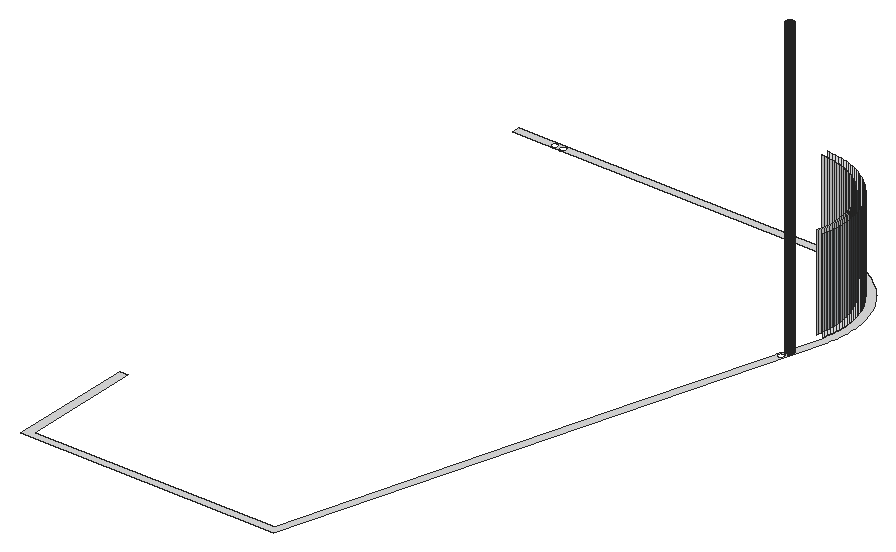
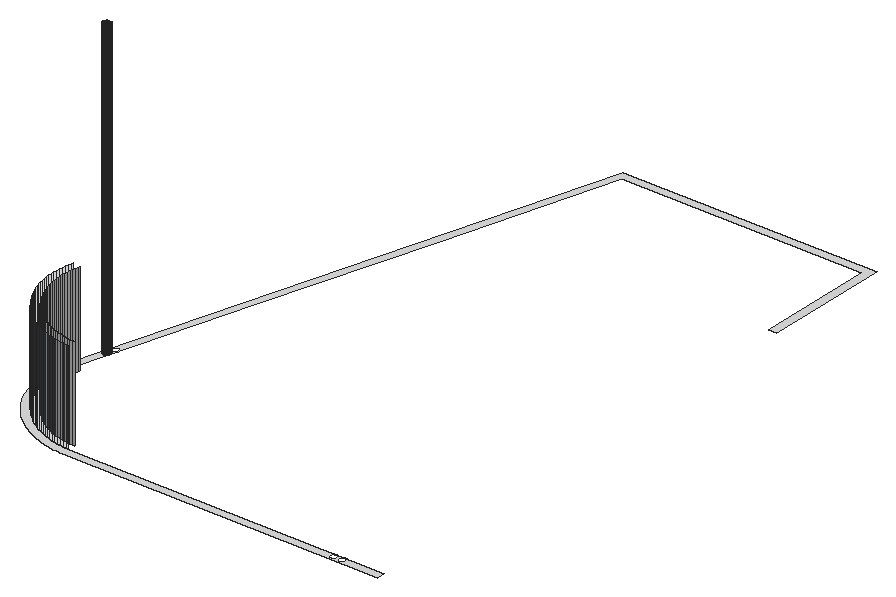
# SketchUp Ruby script. Lengths in inches.
U = 1.inch
M = Sketchup.active_model
def pt(a) = Geom::Point3d.new(a.map { |v| v * U })
def face(e, loops, mat)
  f = e.add_face(loops[0].map { |a| pt(a) })
  loops[1..].each { |l| e.add_face(l.map { |a| pt(a) }).erase! }
  f.material = f.back_material = mat if mat
  f
end
# faces: each face lists its corners as indices into pts; further lists are holes
def faces(e, pts, list, mat = nil) = list.each { |f| face(e, (f[0].is_a?(Array) ? f : [f]).map { |l| l.map { |i| pts[i] } }, mat) }
# xy, xz, yz: faces in a plane at the given z, y or x. An outline is a flat list of corners, or four numbers for a rectangle; further outlines are holes
def ring(l) = l.size == 4 ? [[l[0], l[1]], [l[2], l[1]], [l[2], l[3]], [l[0], l[3]]] : l.each_slice(2).to_a
def flat(e, list, mat, &to3) = list.each { |f| face(e, (f[0].is_a?(Array) ? f : [f]).map { |l| ring(l).map { |u, v| to3.(u, v) } }, mat) }
def xy(e, z, list, mat = nil) = flat(e, list, mat) { |x, y| [x, y, z] }
def xz(e, y, list, mat = nil) = flat(e, list, mat) { |x, z| [x, y, z] }
def yz(e, x, list, mat = nil) = flat(e, list, mat) { |y, z| [x, y, z] }
def lines(e, pts, list) = list.each { |a, b| e.add_line(pt(pts[a]), pt(pts[b])) }
# prism: a flat outline (further loops are holes) pulled along v
def prism(e, loops, v, mat = nil)
  f = face(e, loops, mat); d = Geom::Vector3d.new(v.map { |x| x * U })
  f.pushpull(f.normal.samedirection?(d) ? d.length : -d.length)
end
def box(e, o, s, mat = nil) = prism(e, [[o, [o[0] + s[0], o[1], o[2]], [o[0] + s[0], o[1] + s[1], o[2]], [o[0], o[1] + s[1], o[2]]]], [0, 0, s[2]], mat)
def at(x, y, z, deg = 0) = Geom::Transformation.translation(pt([x, y, z])) * Geom::Transformation.rotation(ORIGIN, Z_AXIS, deg.degrees)
def axes(o, x, y, z) = Geom::Transformation.new([*x, 0, *y, 0, *z, 0, *pt(o).to_a, 1])
def part(name) = M.definitions.add(name)
# library, detail: a bought-in or finely detailed component or shape, given as its bounding box
def library(name, o, s) = part(name).tap { |d| box(d.entities, o, s) }
def detail(e, o, s) = box(e.add_group.entities, o, s)
def put(e, d, t, mat = nil) = e.add_instance(d, t).tap { |i| i.material = mat if mat }
def group(e, t, mat = nil) = e.add_group.tap { |g| g.transformation = t; g.material = mat if mat }.entities
root = M.entities
M.materials.add("Glass_Basic_01").color = [105, 113, 122]
M.materials["Glass_Basic_01"].alpha = 0.25
M.materials.add("M01_Silver_Fog").color = [224, 224, 224]
xy(root,270,[[[210,240,307.76,240,364.95,435.42,365.24,436.52,365.52,437.84,365.76,439.16,365.94,440.5,366.07,441.84,366.16,443.18,366.1875,444.52,366.17,445.87,366.1,447.21,365.98,448.55,365.8,449.89,365.58,451.21,365.3,452.53,364.98,453.84,364.61,455.13,364.18,456.41,363.71,457.67,363.2,458.91,362.63,460.13,362.02,461.33,361.36,462.5,360.69,463.59,360.66,463.65,359.92,464.77,359.13,465.86,358.3,466.92,357.4375,467.95,357.39,468,356.53,468.95,355.59,469.91,354.61,470.83,353.6,471.72,352.55,472.5625,351.47,473.37,350.37,474.13,349.23,474.85,348.07,475.53,346.88,476.16,345.67,476.75,344.44,477.29,343.1875,477.79,341.92,478.23,340.63,478.63,339.33,478.98,338.02,479.28,336.7,479.52,335.37,479.72,334.03,479.87,332.69,479.96,331.55,480,210,480,210,477,331.5,477,332.53,476.97,333.76,476.88,334.99,476.74,336.2,476.5625,337.41,476.34,338.61,476.0625,339.8,475.75,340.98,475.38,342.14,474.97,343.29,474.52,344.41,474.03,345.52,473.49,346.61,472.91,347.67,472.29,348.71,471.63,349.72,470.93,350.71,470.19,351.67,469.42,352.59,468.61,353.49,467.76,354.35,466.89,355.17,465.98,355.18,465.98,355.97,465.03,356.73,464.0625,357.45,463.0625,358.13,462.04,358.13,462.03,358.77,460.99,359.37,459.91,359.93,458.82,360.45,457.7,360.92,456.5625,361.35,455.41,361.74,454.24,362.08,453.06,362.38,451.86,362.63,450.66,362.83,449.44,362.99,448.22,363.1,447,363.17,445.77,363.1875,444.54,363.16,443.31,363.08,442.08,362.96,440.85,362.79,439.63,362.58,438.42,362.32,437.22,362.06,436.22,343.2,371.78,324.34,307.35,305.51,243,213,243,213,288,210,288],[358.91,418.8,358.82,418.81,358.73,418.8125,358.65,418.83,358.5625,418.85,358.48,418.87,358.39,418.9,358.3125,418.9375,358.24,418.98,358.16,419.02,358.09,419.07,357.95,419.18,357.89,419.24,357.83,419.31,357.73,419.45,357.68,419.53,357.64,419.61,357.61,419.6875,357.58,419.77,357.55,419.85,357.54,419.94,357.52,420.03,357.51,420.11,357.51,420.29,357.52,420.38,357.54,420.46,357.55,420.55,357.58,420.64,357.64,420.8,357.68,420.88,357.73,420.95,357.78,421.03,357.83,421.09,357.89,421.16,357.95,421.22,358.09,421.34,358.16,421.38,358.24,421.43,358.3125,421.47,358.39,421.5,358.48,421.53,358.5625,421.56,358.65,421.58,358.73,421.59,358.82,421.6,359,421.6,359.09,421.59,359.17,421.58,359.26,421.56,359.34,421.53,359.43,421.5,359.51,421.47,359.58,421.43,359.66,421.38,359.73,421.34,359.87,421.22,359.93,421.16,359.99,421.09,360.04,421.03,360.09,420.95,360.14,420.88,360.18,420.8,360.24,420.64,360.27,420.55,360.29,420.46,360.3,420.38,360.31,420.29,360.31,420.11,360.3,420.03,360.29,419.94,360.27,419.85,360.24,419.77,360.21,419.6875,360.18,419.61,360.14,419.53,360.09,419.45,359.99,419.31,359.93,419.24,359.87,419.18,359.73,419.07,359.66,419.02,359.58,418.98,359.51,418.9375,359.43,418.9,359.34,418.87,359.26,418.85,359.17,418.83,359.09,418.8125,359,418.81],[359.74,421.95,359.66,421.96,359.57,421.97,359.48,421.99,359.32,422.05,359.23,422.08,359.16,422.12,359.08,422.17,359.01,422.21,358.9375,422.27,358.87,422.33,358.75,422.45,358.7,422.52,358.65,422.6,358.6,422.67,358.5625,422.75,358.53,422.83,358.5,422.91,358.47,423,358.46,423.08,358.44,423.17,358.43,423.26,358.43,423.44,358.44,423.52,358.46,423.61,358.47,423.7,358.53,423.86,358.5625,423.94,358.6,424.02,358.65,424.1,358.75,424.24,358.81,424.31,358.87,424.37,358.9375,424.43,359.01,424.48,359.08,424.53,359.16,424.57,359.23,424.61,359.32,424.65,359.4,424.68,359.48,424.7,359.66,424.74,359.74,424.74,359.83,424.75,359.92,424.74,360.01,424.74,360.09,424.72,360.18,424.7,360.26,424.68,360.35,424.65,360.51,424.57,360.58,424.53,360.72,424.43,360.79,424.37,360.85,424.31,360.91,424.24,361.01,424.1,361.06,424.02,361.1,423.94,361.16,423.78,361.1875,423.7,361.21,423.61,361.22,423.52,361.23,423.44,361.23,423.26,361.21,423.08,361.1875,423,361.16,422.91,361.1,422.75,361.06,422.67,361.01,422.6,360.96,422.52,360.91,422.45,360.79,422.33,360.65,422.21,360.58,422.17,360.51,422.12,360.43,422.08,360.35,422.05,360.26,422.02,360.18,421.99,360.09,421.97,360.01,421.96,359.92,421.95],[228.34,477.03,228.25,477.04,228.17,477.06,228.08,477.08,228,477.11,227.91,477.14,227.84,477.18,227.76,477.22,227.68,477.27,227.54,477.37,227.48,477.43,227.42,477.5,227.36,477.56,227.3125,477.64,227.26,477.71,227.18,477.87,227.15,477.95,227.125,478.03,227.1,478.12,227.09,478.2,227.07,478.29,227.07,478.55,227.08,478.64,227.1,478.73,227.12,478.8125,227.15,478.9,227.18,478.98,227.22,479.06,227.26,479.13,227.31,479.21,227.41,479.35,227.47,479.41,227.61,479.53,227.75,479.63,227.91,479.71,228.07,479.77,228.16,479.79,228.24,479.81,228.33,479.82,228.42,479.82,228.51,479.83,228.59,479.82,228.68,479.81,228.77,479.79,228.85,479.77,228.9375,479.74,229.02,479.71,229.1,479.68,229.18,479.63,229.25,479.59,229.32,479.53,229.39,479.48,229.45,479.42,229.51,479.35,229.57,479.29,229.62,479.22,229.67,479.14,229.71,479.07,229.75,478.99,229.78,478.9,229.81,478.82,229.83,478.74,229.85,478.65,229.86,478.5625,229.87,478.47,229.87,478.39,229.85,478.21,229.83,478.125,229.8125,478.04,229.79,477.96,229.75,477.875,229.72,477.79,229.67,477.72,229.63,477.64,229.58,477.57,229.52,477.5,229.46,477.4375,229.4,477.38,229.33,477.32,229.26,477.27,229.18,477.22,229.11,477.18,229.03,477.14,228.95,477.11,228.86,477.08,228.78,477.06,228.69,477.04,228.6,477.03],[225.03,477.03,224.94,477.04,224.85,477.06,224.77,477.08,224.68,477.11,224.6,477.14,224.52,477.18,224.45,477.22,224.37,477.27,224.23,477.37,224.17,477.43,224.11,477.5,224.05,477.56,224,477.64,223.95,477.71,223.87,477.87,223.84,477.95,223.8125,478.03,223.77,478.2,223.76,478.29,223.76,478.55,223.77,478.64,223.79,478.73,223.81,478.8125,223.84,478.9,223.87,478.98,223.91,479.06,223.95,479.13,223.99,479.21,224.05,479.28,224.1,479.35,224.16,479.41,224.23,479.47,224.29,479.53,224.36,479.58,224.4375,479.63,224.52,479.67,224.6,479.71,224.76,479.77,224.85,479.79,224.93,479.81,225.02,479.82,225.11,479.82,225.19,479.83,225.37,479.81,225.46,479.79,225.54,479.77,225.71,479.71,225.79,479.68,225.86,479.63,225.9375,479.59,226.01,479.53,226.08,479.48,226.14,479.42,226.2,479.35,226.26,479.29,226.3125,479.22,226.36,479.14,226.4,479.07,226.4375,478.99,226.47,478.9,226.5,478.82,226.52,478.74,226.54,478.65,226.55,478.5625,226.55,478.3,226.54,478.21,226.5,478.04,226.47,477.96,226.44,477.875,226.4,477.79,226.36,477.72,226.32,477.64,226.26,477.57,226.21,477.5,226.15,477.4375,226.08,477.38,226.02,477.32,225.95,477.27,225.87,477.22,225.71,477.14,225.55,477.08,225.46,477.06,225.38,477.04,225.29,477.03]]],"M01_Silver_Fog")
xz(root,424.74,[[359.66,270,359.74,384],[359.92,270,360.01,384]],"M01_Silver_Fog")
xz(root,465.98,[[355.17,270,355.18,306]],"Glass_Basic_01")
yz(root,358.13,[[462.03,270,462.04,306]],"Glass_Basic_01")
yz(root,358.43,[[423.26,270,423.35,384],[423.35,270,423.44,384]],"M01_Silver_Fog")
yz(root,361.23,[[423.26,270,423.35,384],[423.35,270,423.44,384]],"M01_Silver_Fog")
p = [[359.23,422.08,270],[359.32,422.05,270],[359.32,422.05,384],[359.23,422.08,384],[360.26,422.02,270],[360.35,422.05,270],
  [360.35,422.05,384],[360.26,422.02,384],[360.43,422.08,270],[360.43,422.08,384],[359.08,422.17,270],[359.16,422.12,270],
  [359.16,422.12,384],[359.08,422.17,384],[360.51,422.12,270],[360.51,422.12,384],[360.58,422.17,270],[360.58,422.17,384],
  [358.9375,422.27,270],[359.01,422.21,270],[359.01,422.21,384],[358.9375,422.27,384],[360.65,422.21,270],[360.65,422.21,384],
  [360.72,422.27,270],[360.72,422.27,384],[358.81,422.39,270],[358.87,422.33,270],[358.87,422.33,384],[358.81,422.39,384],
  [360.79,422.33,270],[360.79,422.33,384],[360.85,422.39,270],[360.85,422.39,384],[358.75,422.45,270],[358.75,422.45,384],
  [360.91,422.45,270],[360.91,422.45,384],[358.65,422.6,270],[358.7,422.52,270],[358.7,422.52,384],[358.65,422.6,384],
  [360.96,422.52,270],[360.96,422.52,384],[361.01,422.6,270],[361.01,422.6,384],[358.6,422.67,270],[358.6,422.67,384],
  [361.06,422.67,270],[361.06,422.67,384],[358.5625,422.75,270],[358.5625,422.75,384],[361.1,422.75,270],[361.1,422.75,384],
  [358.53,422.83,270],[358.53,422.83,384],[358.5,422.91,270],[358.5,422.91,384],[361.13,422.83,270],[361.13,422.83,384],
  [361.16,422.91,270],[361.16,422.91,384],[358.47,423,270],[358.47,423,384],[361.1875,423,270],[361.1875,423,384],
  [358.46,423.08,270],[358.46,423.08,384],[361.21,423.08,270],[361.21,423.08,384],[358.44,423.17,270],[358.44,423.17,384],
  [361.22,423.17,270],[361.22,423.17,384],[358.43,423.26,270],[358.43,423.26,384],[361.23,423.26,270],[361.23,423.26,384],
  [358.44,423.52,270],[358.43,423.44,270],[358.43,423.44,384],[358.44,423.52,384],[361.23,423.44,270],[361.22,423.52,270],
  [361.22,423.52,384],[361.23,423.44,384],[358.46,423.61,270],[358.46,423.61,384],[361.21,423.61,270],[361.21,423.61,384],
  [358.47,423.7,270],[358.47,423.7,384],[361.1875,423.7,270],[361.1875,423.7,384],[358.5,423.78,270],[358.5,423.78,384],
  [361.16,423.78,270],[361.16,423.78,384],[358.53,423.86,270],[358.53,423.86,384],[361.13,423.86,270],[361.13,423.86,384],
  [358.5625,423.94,270],[358.5625,423.94,384],[358.6,424.02,270],[358.6,424.02,384],[361.1,423.94,270],[361.1,423.94,384],
  [361.06,424.02,270],[361.06,424.02,384],[358.65,424.1,270],[358.65,424.1,384],[361.01,424.1,270],[361.01,424.1,384],
  [358.7,424.17,270],[358.7,424.17,384],[360.96,424.17,270],[360.96,424.17,384],[358.75,424.24,270],[358.75,424.24,384],
  [358.81,424.31,270],[358.81,424.31,384],[360.91,424.24,270],[360.91,424.24,384],[360.85,424.31,270],[360.85,424.31,384],
  [358.87,424.37,270],[358.87,424.37,384],[360.79,424.37,270],[360.79,424.37,384],[358.9375,424.43,270],[358.9375,424.43,384],
  [359.01,424.48,270],[359.01,424.48,384],[360.72,424.43,270],[360.72,424.43,384],[360.65,424.48,270],[360.65,424.48,384],
  [359.08,424.53,270],[359.08,424.53,384],[359.16,424.57,270],[359.16,424.57,384],[360.58,424.53,270],[360.51,424.57,270],
  [360.51,424.57,384],[360.58,424.53,384],[359.23,424.61,270],[359.23,424.61,384],[359.32,424.65,270],[359.32,424.65,384],
  [359.4,424.68,270],[359.4,424.68,384],[360.43,424.61,270],[360.35,424.65,270],[360.35,424.65,384],[360.43,424.61,384],
  [360.26,424.68,270],[360.26,424.68,384],[359.48,424.7,270],[359.48,424.7,384],[359.57,424.72,270],[359.57,424.72,384],
  [359.66,424.74,270],[359.66,424.74,384],[359.83,424.75,270],[359.74,424.74,270],[359.74,424.74,384],[359.83,424.75,384],
  [359.92,424.74,270],[359.92,424.74,384],[360.09,424.72,270],[360.01,424.74,270],[360.01,424.74,384],[360.09,424.72,384],
  [360.18,424.7,270],[360.18,424.7,384],[362.06,436.22,270],[362.32,437.22,270],[362.32,437.22,306],[362.06,436.22,306],
  [359.4,437.91,270],[359.17,437.01,270],[359.17,437.01,306],[359.4,437.91,306],[362.58,438.42,270],[362.58,438.42,306],
  [359.63,439,270],[359.63,439,306],[362.79,439.63,270],[362.79,439.63,306],[359.83,440.1,270],[359.83,440.1,306],
  [362.96,440.85,270],[362.96,440.85,306],[359.98,441.21,270],[359.98,441.21,306],[363.08,442.08,270],[363.08,442.08,306],
  [360.09,442.32,270],[360.09,442.32,306],[363.16,443.31,270],[363.16,443.31,306],[360.16,443.43,270],[360.16,443.43,306],
  [363.1875,444.54,270],[363.1875,444.54,306],[360.1875,444.55,270],[360.1875,444.55,306],[360.17,445.67,270],[360.17,445.67,306],
  [363.17,445.77,270],[363.17,445.77,306],[360.11,446.78,270],[360.11,446.78,306],[363.1,447,270],[363.1,447,306],
  [360.01,447.89,270],[360.01,447.89,306],[362.99,448.22,270],[362.99,448.22,306],[359.87,449,270],[359.87,449,306],
  [362.83,449.44,270],[362.83,449.44,306],[359.68,450.1,270],[359.68,450.1,306],[362.63,450.66,270],[362.63,450.66,306],
  [359.45,451.2,270],[359.45,451.2,306],[362.38,451.86,270],[362.38,451.86,306],[359.18,452.28,270],[359.18,452.28,306],
  [362.08,453.06,270],[362.08,453.06,306],[358.875,453.35,270],[358.875,453.35,306],[361.74,454.24,270],[361.74,454.24,306],
  [358.52,454.41,270],[358.52,454.41,306],[361.35,455.41,270],[361.35,455.41,306],[358.13,455.46,270],[358.13,455.46,306],
  [360.92,456.5625,270],[360.92,456.5625,306],[357.7,456.49,270],[357.7,456.49,306],[357.23,457.5,270],[357.23,457.5,306],
  [360.45,457.7,270],[360.45,457.7,306],[356.73,458.5,270],[356.73,458.5,306],[359.93,458.82,270],[359.93,458.82,306],
  [356.18,459.47,270],[356.18,459.47,306],[359.37,459.91,270],[359.37,459.91,306],[355.6,460.43,270],[355.6,460.43,306],
  [358.77,460.99,270],[358.77,460.99,306],[354.98,461.36,270],[354.98,461.36,306],[358.13,462.03,270],[358.13,462.03,306],
  [354.33,462.26,270],[354.33,462.26,306],[358.13,462.04,270],[357.45,463.0625,270],[357.45,463.0625,306],[358.13,462.04,306],
  [353.64,463.14,270],[353.64,463.14,306],[352.92,464,270],[352.92,464,306],[356.73,464.0625,270],[356.73,464.0625,306],
  [352.17,464.83,270],[352.17,464.83,306],[355.97,465.03,270],[355.97,465.03,306],[351.39,465.62,270],[351.39,465.62,306],
  [355.18,465.98,270],[355.18,465.98,306],[350.58,466.39,270],[350.58,466.39,306],[355.17,465.98,270],[354.35,466.89,270],
  [354.35,466.89,306],[355.17,465.98,306],[349.74,467.125,270],[349.74,467.125,306],[353.49,467.76,270],[353.49,467.76,306],
  [348.87,467.83,270],[348.87,467.83,306],[347.97,468.5,270],[347.97,468.5,306],[352.59,468.61,270],[352.59,468.61,306],
  [347.05,469.13,270],[347.05,469.13,306],[351.67,469.42,270],[351.67,469.42,306],[346.11,469.73,270],[346.11,469.73,306],
  [350.71,470.19,270],[350.71,470.19,306],[345.15,470.29,270],[345.15,470.29,306],[349.72,470.93,270],[349.72,470.93,306],
  [344.16,470.82,270],[344.16,470.82,306],[343.16,471.3,270],[343.16,471.3,306],[348.71,471.63,270],[348.71,471.63,306],
  [342.13,471.75,270],[342.13,471.75,306],[347.67,472.29,270],[347.67,472.29,306],[341.09,472.16,270],[341.09,472.16,306],
  [340.04,472.53,270],[340.04,472.53,306],[346.61,472.91,270],[346.61,472.91,306],[338.97,472.86,270],[338.97,472.86,306],
  [337.89,473.15,270],[337.89,473.15,306],[345.52,473.49,270],[345.52,473.49,306],[336.8,473.4,270],[336.8,473.4,306],
  [335.71,473.6,270],[335.71,473.6,306],[344.41,474.03,270],[344.41,474.03,306],[334.6,473.77,270],[334.6,473.77,306],
  [333.49,473.89,270],[333.49,473.89,306],[332.38,473.97,270],[332.38,473.97,306],[331.45,474,270],[331.45,474,306],
  [343.29,474.52,270],[343.29,474.52,306],[342.14,474.97,270],[342.14,474.97,306],[340.98,475.38,270],[340.98,475.38,306],
  [339.8,475.75,270],[339.8,475.75,306],[338.61,476.0625,270],[338.61,476.0625,306],[337.41,476.34,270],[337.41,476.34,306],
  [336.2,476.5625,270],[336.2,476.5625,306],[334.99,476.74,270],[334.99,476.74,306],[333.76,476.88,270],[333.76,476.88,306],
  [332.53,476.97,270],[332.53,476.97,306],[331.5,477,270],[331.5,477,306]]
faces(root,p,[[0,1,2,3],[4,5,6,7],[5,8,9,6],[10,11,12,13],[11,0,3,12],[8,14,15,9],[14,16,17,15],[18,19,20,21],
  [19,10,13,20],[16,22,23,17],[22,24,25,23],[26,27,28,29],[27,18,21,28],[24,30,31,25],[30,32,33,31],[34,26,29,35],
  [32,36,37,33],[38,39,40,41],[39,34,35,40],[36,42,43,37],[42,44,45,43],[46,38,41,47],[44,48,49,45],[50,46,47,51],
  [48,52,53,49],[54,50,51,55],[56,54,55,57],[52,58,59,53],[58,60,61,59],[62,56,57,63],[60,64,65,61],[66,62,63,67],
  [64,68,69,65],[70,66,67,71],[68,72,73,69],[74,70,71,75],[72,76,77,73],[78,79,80,81],[82,83,84,85],[86,78,81,87],
  [83,88,89,84],[90,86,87,91],[88,92,93,89],[94,90,91,95],[92,96,97,93],[98,94,95,99],[96,100,101,97],[102,98,99,103],
  [104,102,103,105],[100,106,107,101],[106,108,109,107],[110,104,105,111],[108,112,113,109],[114,110,111,115],[112,116,117,113],[118,114,115,119],
  [120,118,119,121],[116,122,123,117],[122,124,125,123],[126,120,121,127],[124,128,129,125],[130,126,127,131],[132,130,131,133],[128,134,135,129],
  [134,136,137,135],[138,132,133,139],[140,138,139,141],[142,143,144,145],[136,142,145,137],[146,140,141,147],[148,146,147,149],[150,148,149,151],
  [152,153,154,155],[153,156,157,154],[143,152,155,144],[158,150,151,159],[160,158,159,161],[162,160,161,163],[164,165,166,167],[168,164,167,169],
  [170,171,172,173],[174,170,173,175],[156,174,175,157],[180,181,182,183],[186,180,183,187],[190,186,187,191],[194,190,191,195],[198,194,195,199],
  [202,198,199,203],[206,202,203,207],[208,206,207,209],[212,208,209,213],[216,212,213,217],[220,216,217,221],[224,220,221,225],[228,224,225,229],
  [232,228,229,233],[236,232,233,237],[240,236,237,241],[244,240,241,245],[248,244,245,249],[250,248,249,251],[254,250,251,255],[258,254,255,259],
  [262,258,259,263],[266,262,263,267],[270,266,267,271],[276,270,271,277],[278,276,277,279],[282,278,279,283],[286,282,283,287],[290,286,287,291],
  [296,290,291,297],[300,296,297,301],[302,300,301,303],[306,302,303,307],[310,306,307,311],[314,310,311,315],[318,314,315,319],[320,318,319,321],
  [324,320,321,325],[328,324,325,329],[330,328,329,331],[334,330,331,335],[336,334,335,337],[340,336,337,341],[342,340,341,343],[346,342,343,347],
  [348,346,347,349],[350,348,349,351],[352,350,351,353]],"M01_Silver_Fog")
faces(root,p,[[176,177,178,179],[177,184,185,178],[184,188,189,185],[188,192,193,189],[192,196,197,193],[196,200,201,197],[200,204,205,201],[204,210,211,205],
  [210,214,215,211],[214,218,219,215],[218,222,223,219],[222,226,227,223],[226,230,231,227],[230,234,235,231],[234,238,239,235],[238,242,243,239],
  [242,246,247,243],[246,252,253,247],[252,256,257,253],[256,260,261,257],[260,264,265,261],[264,268,269,265],[272,273,274,275],[273,280,281,274],
  [280,284,285,281],[284,288,289,285],[292,293,294,295],[293,298,299,294],[298,304,305,299],[304,308,309,305],[308,312,313,309],[312,316,317,313],
  [316,322,323,317],[322,326,327,323],[326,332,333,327],[332,338,339,333],[338,344,345,339],[344,354,355,345],[354,356,357,355],[356,358,359,357],
  [358,360,361,359],[360,362,363,361],[362,364,365,363],[364,366,367,365],[366,368,369,367],[368,370,371,369],[370,372,373,371],[372,374,375,373]],"Glass_Basic_01")
